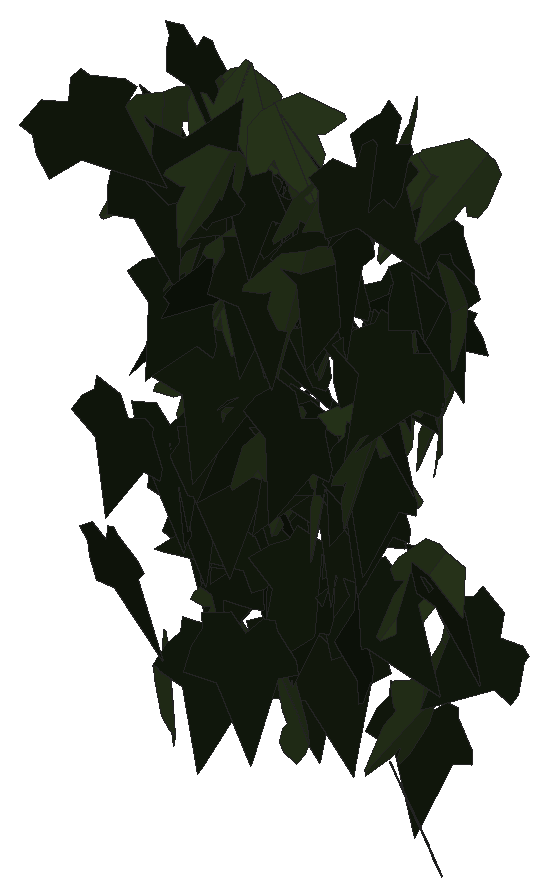
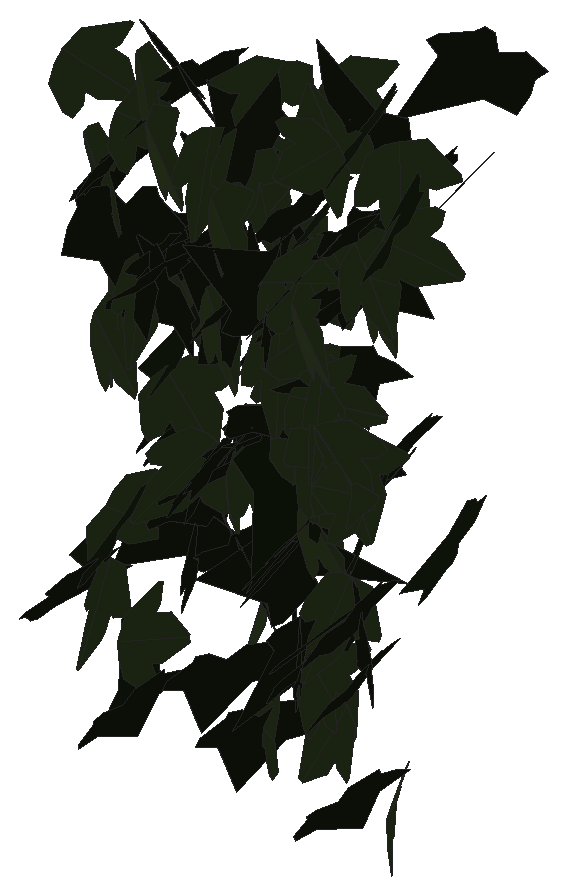
# SketchUp Ruby script. Lengths in inches.
U = 1.inch
M = Sketchup.active_model
def pt(a) = Geom::Point3d.new(a.map { |v| v * U })
def face(e, loops, mat)
  f = e.add_face(loops[0].map { |a| pt(a) })
  loops[1..].each { |l| e.add_face(l.map { |a| pt(a) }).erase! }
  f.material = f.back_material = mat if mat
  f
end
# faces: each face lists its corners as indices into pts; further lists are holes
def faces(e, pts, list, mat = nil) = list.each { |f| face(e, (f[0].is_a?(Array) ? f : [f]).map { |l| l.map { |i| pts[i] } }, mat) }
# xy, xz, yz: faces in a plane at the given z, y or x. An outline is a flat list of corners, or four numbers for a rectangle; further outlines are holes
def ring(l) = l.size == 4 ? [[l[0], l[1]], [l[2], l[1]], [l[2], l[3]], [l[0], l[3]]] : l.each_slice(2).to_a
def flat(e, list, mat, &to3) = list.each { |f| face(e, (f[0].is_a?(Array) ? f : [f]).map { |l| ring(l).map { |u, v| to3.(u, v) } }, mat) }
def xy(e, z, list, mat = nil) = flat(e, list, mat) { |x, y| [x, y, z] }
def xz(e, y, list, mat = nil) = flat(e, list, mat) { |x, z| [x, y, z] }
def yz(e, x, list, mat = nil) = flat(e, list, mat) { |y, z| [x, y, z] }
def lines(e, pts, list) = list.each { |a, b| e.add_line(pt(pts[a]), pt(pts[b])) }
# prism: a flat outline (further loops are holes) pulled along v
def prism(e, loops, v, mat = nil)
  f = face(e, loops, mat); d = Geom::Vector3d.new(v.map { |x| x * U })
  f.pushpull(f.normal.samedirection?(d) ? d.length : -d.length)
end
def box(e, o, s, mat = nil) = prism(e, [[o, [o[0] + s[0], o[1], o[2]], [o[0] + s[0], o[1] + s[1], o[2]], [o[0], o[1] + s[1], o[2]]]], [0, 0, s[2]], mat)
def at(x, y, z, deg = 0) = Geom::Transformation.translation(pt([x, y, z])) * Geom::Transformation.rotation(ORIGIN, Z_AXIS, deg.degrees)
def axes(o, x, y, z) = Geom::Transformation.new([*x, 0, *y, 0, *z, 0, *pt(o).to_a, 1])
def part(name) = M.definitions.add(name)
# library, detail: a bought-in or finely detailed component or shape, given as its bounding box
def library(name, o, s) = part(name).tap { |d| box(d.entities, o, s) }
def detail(e, o, s) = box(e.add_group.entities, o, s)
def put(e, d, t, mat = nil) = e.add_instance(d, t).tap { |i| i.material = mat if mat }
def group(e, t, mat = nil) = e.add_group.tap { |g| g.transformation = t; g.material = mat if mat }.entities
root = M.entities
M.materials.add("efeu1").color = [18, 25, 13]
M.materials.add("efeu2").color = [43, 57, 29]
c1 = part("ivyleaf_9")
p = [[1.54,2.16,1.25],[1.36,2.04,1.19],[-0.21,0.99,0.68],[-0.71,1.11,0.82],[-0.85,0.86,0.67],[-0.8,0.17,0.21],
  [-0.9,-0.01,0.1],[-0.67,-0.16,-0.02],[-0.08,-0.08,-0.05],[-0.03,-0.6,-0.4],[0.65,-0.88,-0.66],[0.83,-0.6,-0.49],
  [1.29,-0.42,-0.43],[1.8125,-0.07,-0.26],[1.21,0.44,0.15]]
faces(c1.entities,p,[[0,1,2,3,4,5,6,7,8,9,10,11,12,13,14]],"efeu1")
c2 = part("ivyleaf_10")
p = [[0,0.5,-0.03],[-0.0625,2.02,-0.43],[-0.19,2.01,-0.46],[-0.54,1.05,-0.29],[-0.52,0.625,-0.18],[-0.83,0.76,-0.28],
  [-1.16,0.64,-0.33],[-1.15,0.33,-0.24],[-0.77,-0.39,0.02],[-0.3,-0.51,0.16],[0.04,-0.48,0.23],[-0.02,2.01,-0.4375],
  [-0.06,2.01,-0.43],[0.04,-0.49,0.23],[0.67,-0.49,0.14],[1.38,0.36,-0.2],[1.375,0.51,-0.24],[0.81,0.65,-0.19],
  [0.62,0.59,-0.15],[0.6,1.09,-0.28],[0.5,1.23,-0.31]]
faces(c2.entities,p,[[0,1,2,3,4,5,6,7,8,9,10],[11,12,0,13,14,15,16,17,18,19,20]],"efeu2")
put(root,c1,axes([25.35,218.63,239.0625],[-0.02983,-0.43524,0.24429],[0.04178,-0.24605,-0.43326],[0.49736,-0.00544,0.05105]))
put(root,c1,axes([26.66,219.1875,236.42],[-0.03539,-0.49289,-0.07618],[0.00862,0.07576,-0.49415],[0.49867,-0.03629,0.00314]))
put(root,c1,axes([23.63,219.78,242.13],[0.0301,-0.17717,-0.46659],[0.17324,0.44208,-0.15669],[0.46806,-0.15222,0.088]))
put(root,c1,axes([23.73,220.33,236.12],[0.31137,-0.39107,0.01073],[0.00566,-0.0092,-0.49988],[0.39118,0.31142,-0.0013]))
put(root,c2,axes([25.15,220.57,241.49],[-0.10252,-0.41524,0.25898],[0.00106,-0.26479,-0.42413],[0.48938,-0.08641,0.05517]))
put(root,c1,axes([26.23,220.71,238.46],[-0.03375,-0.44728,0.22091],[-0.02017,-0.22001,-0.44854],[0.49845,-0.03918,-0.00319]))
put(root,c1,axes([24.49,220.8,239.48],[-0.09699,-0.39948,0.28462],[0.00802,-0.29138,-0.40624],[0.49044,-0.07424,0.06293]))
put(root,c2,axes([27.18,220.75,238.42],[0.12932,-0.47512,0.08681],[0.02867,-0.08216,-0.49237],[0.48213,0.13233,0.00599]))
put(root,c1,axes([24.77,220.88,239.78],[-0.19271,0.20278,-0.41442],[0.15334,-0.39544,-0.2648],[-0.43514,-0.22915,0.09022]))
put(root,c2,axes([26.21,220.72,234.4],[-0.27564,0.40178,0.11222],[0.05993,-0.09497,0.48723],[0.41283,0.28205,0.0042]))
put(root,c1,axes([24.68,220.66,240.95],[-0.29486,0.11771,0.38627],[0.32637,-0.21217,0.31379],[0.23779,0.43718,0.04829]))
put(root,c1,axes([23.86,220.87,240.86],[0.14501,-0.4724,-0.07619],[-0.0184,0.07405,-0.49414],[0.47816,0.14612,0.00409]))
put(root,c1,axes([25.46,221.02,240.13],[0.02443,-0.49877,-0.02513],[0.00013,0.02517,-0.49937],[0.4994,0.0244,0.00136]))
put(root,c1,axes([24.08,221.03,237.46],[0.08033,-0.49324,0.01627],[0.00432,-0.01578,-0.49973],[0.49349,0.08043,0.00173]))
put(root,c2,axes([26.08,220.93,240.37],[-0.16357,-0.46773,0.06691],[-0.01401,-0.06597,-0.49543],[0.47228,-0.16395,0.00847]))
put(root,c1,axes([24.22,221.18,236.91],[0.12978,-0.47196,0.10201],[0.03499,-0.09617,-0.48942],[0.48159,0.13417,0.00806]))
put(root,c2,axes([24.23,221.17,239.63],[0.17879,-0.44818,0.13103],[0.05942,-0.11733,-0.48239],[0.46315,0.18807,0.01131]))
put(root,c1,axes([27.42,221.36,233.38],[0.01671,-0.17373,0.46855],[0.17773,-0.43609,-0.16804],[0.46705,0.17217,0.04718]))
put(root,c1,axes([24.75,221.26,238.5],[-0.33814,-0.34889,-0.11805],[0.07847,0.08833,-0.48584],[0.35986,-0.34709,-0.00498]))
put(root,c1,axes([26.16,221.4,240.21],[-0.06605,-0.46204,0.17931],[0.0194,-0.18317,-0.46484],[0.49524,-0.05445,0.04212]))
put(root,c1,axes([24.94,221.4,240.99],[0.06278,-0.45965,0.18649],[0.04131,-0.18248,-0.46367],[0.49432,0.07362,0.01506]))
put(root,c2,axes([25.57,220.97,237.92],[-0.09162,-0.41667,-0.26075],[0.09249,0.24589,-0.42542],[0.48275,-0.12619,0.03202]))
put(root,c1,axes([24.05,221.45,236.81],[0.18367,-0.08835,-0.45657],[0.39833,-0.22345,0.20348],[-0.24,-0.43848,-0.01169]))
put(root,c1,axes([27.24,221.48,239.33],[-0.27611,-0.39962,0.1186],[-0.03244,-0.12122,-0.484],[0.41558,-0.27497,0.04101]))
put(root,c1,axes([24.68,221.33,237.26],[-0.17962,-0.42691,-0.18836],[0.0667,0.17627,-0.46312],[0.46183,-0.1915,-0.00637]))
put(root,c1,axes([26.55,221.56,235.24],[-0.01666,-0.01975,0.49933],[-0.05749,-0.49622,-0.02154],[0.4964,-0.05813,0.01426]))
put(root,c1,axes([25.88,221.6,235.93],[-0.27009,-0.39238,0.15195],[-0.02691,-0.16408,-0.47154],[0.41991,-0.2629,0.06751]))
put(root,c1,axes([25.93,221.47,235.87],[-0.39286,0.07543,-0.29996],[0.29704,-0.04312,-0.39988],[-0.0862,-0.49239,-0.01093]))
put(root,c1,axes([26.57,221.68,237.3],[0.01421,-0.4652,0.18273],[-0.0089,-0.18301,-0.46522],[0.49972,0.00997,-0.01348]))
put(root,c1,axes([26.61,221.33,241.61],[0.14423,-0.39844,-0.26542],[0.05547,0.28924,-0.40406],[0.47552,0.08711,0.12763]))
put(root,c1,axes([25.27,221.59,237.86],[0.01852,0.15839,-0.47389],[-0.02631,-0.47325,-0.1592],[-0.49896,0.03083,-0.00919]))
put(root,c1,axes([24.125,221.78,239.81],[-0.16881,-0.38022,0.27738],[-0.06344,-0.27361,-0.41366],[0.46635,-0.17485,0.04413]))
put(root,c1,axes([26.18,221.57,240.52],[-0.2331,-0.11474,-0.4272],[0.43752,0.0113,-0.24176],[0.06513,-0.48653,0.09513]))
put(root,c2,axes([24.85,221.73,237.4],[-0.09911,-0.29988,-0.38762],[-0.06902,-0.38298,0.31394],[-0.48519,0.11574,0.03452]))
put(root,c2,axes([23.66,221.41,241.44],[-0.25954,-0.42723,-0.01066],[0.00494,0.00947,-0.49989],[0.42733,-0.25959,-0.00069]))
put(root,c2,axes([25.52,221.3,241.88],[0.24173,0.40483,0.16638],[0.08051,0.14569,-0.47148],[-0.43021,0.25473,0.00525]))
put(root,c2,axes([24.67,221.69,239.82],[0.02007,-0.40477,0.29284],[0.05491,-0.28952,-0.40394],[0.49657,0.04837,0.03283]))
put(root,c1,axes([24.67,221.75,239.51],[0.01357,-0.47632,0.15145],[0.01878,-0.15092,-0.47631],[0.49946,0.01862,0.01379]))
put(root,c2,axes([23.47,221.6875,240.61],[0.12444,0.295,-0.38404],[-0.24885,-0.3012,-0.31201],[-0.41543,0.2688,0.07186]))
put(root,c1,axes([26.88,221.61,241.91],[-0.46778,0.08609,-0.15417],[0.15109,-0.03079,-0.47563],[-0.09139,-0.49157,0.00279]))
put(root,c1,axes([26.52,221.8125,237.54],[0.00064,-0.4805,0.13827],[-0.00869,-0.13826,-0.48043],[0.49992,-0.00179,-0.00852]))
put(root,c2,axes([27.03,221.88,234.4],[0.04071,-0.15738,0.47284],[0.11456,-0.45875,-0.16255],[0.48499,0.12158,-0.00129]))
put(root,c1,axes([25.12,221.6875,236.22],[-0.39202,-0.02598,0.30927],[-0.30849,-0.02196,-0.39288],[0.034,-0.49884,0.00119]))
put(root,c2,axes([24.53,221.44,241.26],[0.47028,0.1039,-0.13431],[0.13111,0.02912,0.48162],[0.1079,-0.48822,0.00014]))
put(root,c1,axes([27.4375,221.62,240.36],[0.11606,-0.46172,-0.15278],[-0.04796,0.14544,-0.47597],[0.48397,0.12514,-0.01053]))
put(root,c1,axes([26.59,221.54,235.99],[-0.05094,-0.2483,-0.43099],[0.30039,0.32996,-0.2256],[0.39645,-0.28191,0.11556]))
put(root,c2,axes([25.64,221.88,236.94],[0.08657,-0.21562,0.44273],[0.31058,-0.32494,-0.21898],[0.38216,0.31292,0.07767]))
put(root,c1,axes([25.4,221.82,241.25],[0.12554,-0.26039,0.40797],[0.25912,-0.31981,-0.28386],[0.40877,0.2827,0.05464]))
put(root,c1,axes([25.5,221.95,237.52],[-0.23863,-0.41479,0.14494],[-0.06516,-0.1297,-0.47847],[0.43452,-0.24725,0.00785]))
put(root,c1,axes([26.65,221.51,239.39],[0.11416,-0.3332,-0.35489],[-0.04117,0.3566,-0.34805],[0.48505,0.10869,0.05398]))
put(root,c2,axes([25.38,221.82,237.22],[-0.09342,-0.45901,0.17489],[0.01447,-0.18052,-0.46605],[0.49098,-0.08201,0.04701]))
put(root,c1,axes([23.375,221.89,240.87],[0.20771,-0.38741,0.23827],[0.11774,-0.20721,-0.43955],[0.43931,0.2387,0.00515]))
put(root,c2,axes([24.7,221.94,240.07],[0.00875,0.26367,-0.42474],[-0.14633,-0.40485,-0.25433],[-0.47803,0.12876,0.07008]))
put(root,c2,axes([24.51,221.89,236.88],[0.13618,-0.43237,0.21097],[0.06169,-0.20175,-0.45331],[0.47713,0.14949,-0.00161]))
put(root,c2,axes([25.75,221.58,240.9375],[-0.056,-0.45769,-0.19336],[0.03246,0.1908,-0.46102],[0.49579,-0.06419,0.00834]))
put(root,c1,axes([23.79,221.89,241.97],[0.20018,-0.44779,0.09702],[0.02967,-0.09298,-0.49038],[0.45722,0.20208,-0.01065]))
put(root,c2,axes([27.875,221.54,240.19],[0.2432,-0.20633,-0.38507],[-0.25597,0.28984,-0.31697],[0.35402,0.35131,0.03535]))
put(root,c2,axes([25.16,221.92,239.02],[0.21757,-0.39151,0.22223],[0.12805,-0.18281,-0.44742],[0.43159,0.2516,0.02071]))
put(root,c1,axes([24.3,221.77,240.49],[0.11289,-0.44053,-0.20782],[0.07037,0.22584,-0.44051],[0.48198,0.0702,0.11299]))
put(root,c1,axes([26.32,221.91,238.49],[0.26723,-0.41019,0.10163],[0.04602,-0.09128,-0.48944],[0.42008,0.27094,-0.01103]))
put(root,c2,axes([26.92,222.11,241.2],[-0.08027,-0.27764,0.40801],[0.12002,-0.41194,-0.2567],[0.4787,0.05673,0.13277]))
put(root,c2,axes([27.66,222.1,241.67],[-0.1471,-0.28796,0.38137],[-0.01419,-0.39622,-0.30464],[0.47766,-0.10045,0.1084]))
put(root,c2,axes([24.35,222.13,238.5],[-0.10805,-0.15717,0.46219],[-0.10073,-0.45601,-0.17862],[0.47768,-0.13171,0.06688]))
put(root,c1,axes([27.14,222.11,240.7],[0.01515,-0.47641,0.15101],[0.00079,-0.15106,-0.47664],[0.49977,0.01468,-0.00382]))
put(root,c2,axes([26.36,222.01,237.94],[-0.26144,-0.35066,0.24225],[-0.0489,-0.25764,-0.42571],[0.42339,-0.24628,0.10042]))
put(root,c1,axes([24.79,222.03,236.35],[0.11663,-0.48208,0.06324],[0.01332,-0.06185,-0.49598],[0.48602,0.11738,-0.00158]))
put(root,c2,axes([23.98,221.95,237.77],[-0.18647,-0.44606,0.1275],[-0.01698,-0.13076,-0.4823],[0.46362,-0.1842,0.03362]))
put(root,c1,axes([26.03,222.11,236.77],[-0.14644,-0.47719,0.02906],[-0.00598,-0.02856,-0.49915],[0.47804,-0.14653,0.00266]))
put(root,c1,axes([24.75,221.82,236.1875],[0.41695,-0.14198,0.23663],[0.2222,-0.08149,-0.44044],[0.16363,0.47244,-0.00485]))
put(root,c2,axes([27.49,221.7,238.59],[0.27124,-0.33004,-0.25981],[-0.06409,0.27313,-0.41388],[0.41511,0.25782,0.10586]))
put(root,c1,axes([24.54,222.18,240.43],[0.0461,-0.43841,0.23594],[0.08199,-0.22703,-0.43788],[0.49107,0.07906,0.05096]))
put(root,c2,axes([24.23,222.09,235.02],[-0.01383,-0.44221,0.23294],[0.04617,-0.23316,-0.43989],[0.49767,0.00934,0.04728]))
put(root,c2,axes([24.33,221.94,241.59],[-0.34092,0.02845,-0.36464],[0.33714,-0.16882,-0.32838],[-0.1418,-0.46978,0.09592]))
put(root,c2,axes([26.05,221.8,240.96],[-0.10104,-0.46521,-0.15289],[0.06599,0.14175,-0.47492],[0.48522,-0.11615,0.03275]))
put(root,c2,axes([27.09,222.13,236.19],[0.1584,0.28306,-0.3805],[-0.17056,-0.34032,-0.32418],[-0.44251,0.2325,-0.01126]))
put(root,c2,axes([23.59,221.61,233.29],[-0.13357,0.26505,-0.40238],[-0.1737,0.36299,0.29676],[0.44943,0.21907,-0.00489]))
put(root,c1,axes([27.22,221.82,239.8],[0.25473,0.27058,-0.33452],[-0.23623,-0.23696,-0.37155],[-0.3596,0.34733,0.00712]))
put(root,c1,axes([25.66,221.99,234.68],[-0.07286,-0.44565,-0.21467],[0.05937,0.20754,-0.451],[0.49109,-0.09121,0.02268]))
put(root,c1,axes([25.53,222.06,239.22],[0.25834,-0.04941,-0.42523],[0.42806,0.02425,0.25725],[-0.0048,-0.49696,0.05483]))
put(root,c1,axes([26.65,222.3,239.28],[-0.20628,-0.39666,0.22385],[-0.00326,-0.24445,-0.43616],[0.45545,-0.1814,0.09826]))
put(root,c2,axes([23.62,222.08,240.5],[-0.03974,-0.47517,0.15046],[0.01073,-0.15172,-0.4763],[0.4983,-0.03463,0.02225]))
put(root,c1,axes([24.63,222.1875,239.45],[-0.02185,-0.4985,0.03197],[0.00371,-0.03216,-0.49895],[0.49951,-0.02157,0.00511]))
put(root,c1,axes([25.61,222,237.4],[0.16061,-0.44579,-0.1596],[-0.04438,0.15362,-0.47374],[0.47142,0.16634,0.00978]))
put(root,c2,axes([24.15,221.97,234.46],[-0.42144,0.19539,-0.18497],[0.16134,-0.09155,-0.46431],[-0.21531,-0.45104,0.01412]))
put(root,c2,axes([26.9,221.9,239.1],[-0.05021,-0.46448,-0.17814],[0.04385,0.17422,-0.46661],[0.49554,-0.06248,0.02324]))
put(root,c1,axes([26.37,222.14,239.34],[-0.16278,-0.07036,-0.46749],[0.46685,0.054,-0.17069],[0.07451,-0.49207,0.04811]))
put(root,c1,axes([24.43,222.27,235.01],[-0.00901,0.06475,0.49571],[0.07729,-0.48965,0.06536],[0.49391,0.0778,-0.00119]))
put(root,c1,axes([25.32,222.31,239.5625],[0.01491,-0.47958,0.14065],[0.01871,-0.14008,-0.47961],[0.49943,0.01956,0.01377]))
put(root,c2,axes([25.71,222.11,239.1875],[0.12143,-0.48424,0.02762],[-0.00328,-0.02929,-0.49913],[0.48502,0.12104,-0.01029]))
put(root,c1,axes([25.74,222.39,237.21],[-0.0106,-0.43124,0.25283],[-0.01331,-0.25255,-0.43132],[0.49971,-0.01587,-0.00612]))
put(root,c1,axes([24.5,222.08,240.04],[0.24324,-0.42408,-0.10483],[-0.01466,0.112,-0.48708],[0.4366,0.24002,0.04205]))
put(root,c1,axes([25.35,221.8125,239.34],[0.00594,-0.03912,0.49843],[-0.18821,0.46162,0.03848],[-0.46319,-0.18808,-0.00924]))
put(root,c2,axes([24.14,222.14,237.32],[-0.49813,0.03769,0.02123],[0.01939,-0.02472,0.49901],[0.03867,0.49796,0.02317]))
put(root,c1,axes([24.79,222.36,238.41],[-0.28659,-0.40758,0.04183],[-0.03023,-0.02988,-0.49819],[0.4086,-0.28808,-0.00751]))
put(root,c1,axes([23.72,222.39,233.76],[-0.095,-0.48677,0.0635],[0.01025,-0.06663,-0.49543],[0.49078,-0.09283,0.02264]))
put(root,c2,axes([27.12,222.3,238.52],[0.13357,-0.44394,0.18729],[0.05471,-0.17913,-0.46359],[0.47871,0.14433,0.00072]))
put(root,c2,axes([26.7,222.13,241.86],[0.19105,-0.45572,-0.07627],[-0.01457,0.07655,-0.49389],[0.46183,0.19094,0.01597]))
put(root,c1,axes([26.97,222.3,236.03],[0.26417,-0.41072,0.10734],[0.05568,-0.09181,-0.48833],[0.42085,0.26996,-0.00277]))
put(root,c2,axes([25.47,222.3,240.53],[0.16392,-0.45466,0.12811],[0.04494,-0.11998,-0.48331],[0.47023,0.16996,0.00153]))
put(root,c1,axes([23.46,222.32,236.05],[-0.15358,0.02356,-0.47524],[0.46896,-0.07703,-0.15537],[-0.08054,-0.49347,0.00156]))
put(root,c2,axes([24.49,221.98,238.91],[0.09923,0.4526,0.1879],[0.03927,0.18375,-0.46335],[-0.48848,0.10671,0.00092]))
put(root,c1,axes([24.64,222.46,239.89],[-0.00009,-0.0335,-0.49888],[0.44096,-0.23517,0.01571],[-0.2357,-0.43997,0.02959]))
put(root,c2,axes([26.36,222.34,241.21],[0.23678,-0.41365,0.1511],[0.06676,-0.13586,-0.47653],[0.43529,0.24584,-0.00911]))
put(root,c2,axes([24.02,222.25,238.19],[0.44512,0.11963,-0.19379],[-0.18614,-0.05401,-0.4609],[-0.13121,0.48246,-0.00355]))
put(root,c2,axes([24.44,222.56,240.15],[-0.11871,-0.15313,0.46093],[0.07224,-0.47479,-0.13912],[0.4803,0.03356,0.13485]))
put(root,c1,axes([24.4,221.93,235.5],[0.13175,-0.16981,-0.45145],[-0.13517,0.43624,-0.20354],[0.463,0.17568,0.06904]))
put(root,c1,axes([24.12,222.54,235.44],[-0.05941,-0.45297,0.20319],[0.00405,-0.20508,-0.45599],[0.49644,-0.05254,0.02804]))
put(root,c1,axes([26.72,222.47,233.97],[-0.04177,-0.49548,0.05252],[-0.00354,-0.05241,-0.49723],[0.49824,-0.04191,0.00087]))
put(root,c2,axes([23.98,222.02,236.09],[-0.12914,-0.38038,-0.29771],[0.11298,0.27583,-0.40144],[0.46964,-0.17096,0.01471]))
put(root,c2,axes([24.1875,222.11,238.69],[0.06996,-0.45391,-0.19766],[0.03049,0.20319,-0.45583],[0.49414,0.05173,0.05611]))
put(root,c2,axes([24.62,222.46,234.33],[0.04829,-0.11204,0.48489],[0.44671,-0.20497,-0.09185],[0.21935,0.44208,0.0803]))
put(root,c2,axes([25.98,222.06,237.19],[-0.22035,-0.25543,-0.36905],[0.27462,0.24846,-0.33594],[0.35501,-0.35075,0.0308]))
put(root,c1,axes([24.6,222.21,238.67],[0.29817,-0.35263,-0.1917],[-0.06532,0.19299,-0.45661],[0.39601,0.29734,0.06902]))
put(root,c2,axes([24.2,222.45,239.74],[0.24792,-0.39922,0.17076],[0.07863,-0.15211,-0.46977],[0.42703,0.25979,-0.01264]))
put(root,c1,axes([23.49,222.56,235.35],[0.04556,-0.47928,0.13497],[0.02081,-0.13359,-0.48138],[0.49748,0.04948,0.00777]))
put(root,c2,axes([23.85,222,237.4375],[0.14128,-0.25402,0.40683],[-0.15623,0.37661,0.28941],[-0.45347,-0.20889,0.02704]))
put(root,c1,axes([24.42,222.39,236.86],[0.19708,-0.45555,-0.06026],[0.00227,0.06654,-0.49555],[0.45951,0.19505,0.0283]))
put(root,c1,axes([27.55,222.7,235.18],[-0.22455,-0.33018,0.30093],[-0.07602,-0.30366,-0.38989],[0.44023,-0.22085,0.08617]))
put(root,c1,axes([24.87,222.39,234.41],[-0.08709,-0.44112,-0.21869],[0.05988,0.21095,-0.44935],[0.4887,-0.10446,0.01609]))
put(root,c1,axes([23.51,222.57,236.2],[0.03663,-0.49341,0.07216],[-0.00913,-0.073,-0.49456],[0.49857,0.03492,-0.01435]))
put(root,c2,axes([24.67,222.27,239.16],[-0.14589,-0.4692,-0.09254],[0.01709,0.09157,-0.49125],[0.47794,-0.1465,-0.01068]))
put(root,c2,axes([27.24,222.125,235.21],[0.07054,-0.39667,-0.2961],[0.06288,0.30385,-0.39207],[0.49099,0.01808,0.09275]))
put(root,c1,axes([23.97,222.7,235.8],[-0.14457,-0.40768,0.25079],[0.03122,-0.26945,-0.42002],[0.47762,-0.10579,0.10337]))
put(root,c1,axes([24.8,221.9375,237.28],[0.05432,0.42388,0.25956],[0.0237,0.2586,-0.42728],[-0.49647,0.05872,0.00801]))
put(root,c1,axes([24.78,222.07,239.64],[-0.06374,-0.01325,0.49574],[0.45884,0.18806,0.06403],[-0.18816,0.4631,-0.01181]))
